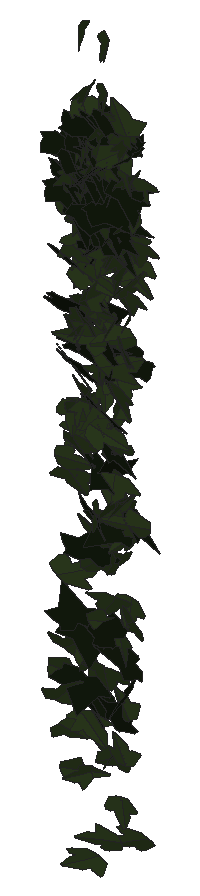
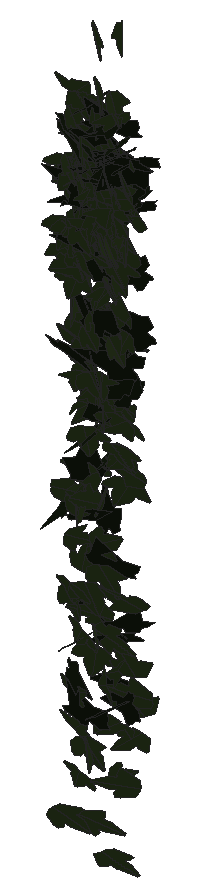
# SketchUp Ruby script. Lengths in millimetres.
U = 1.mm
M = Sketchup.active_model
def pt(a) = Geom::Point3d.new(a.map { |v| v * U })
def face(e, loops, mat)
  f = e.add_face(loops[0].map { |a| pt(a) })
  loops[1..].each { |l| e.add_face(l.map { |a| pt(a) }).erase! }
  f.material = f.back_material = mat if mat
  f
end
# faces: each face lists its corners as indices into pts; further lists are holes
def faces(e, pts, list, mat = nil) = list.each { |f| face(e, (f[0].is_a?(Array) ? f : [f]).map { |l| l.map { |i| pts[i] } }, mat) }
# xy, xz, yz: faces in a plane at the given z, y or x. An outline is a flat list of corners, or four numbers for a rectangle; further outlines are holes
def ring(l) = l.size == 4 ? [[l[0], l[1]], [l[2], l[1]], [l[2], l[3]], [l[0], l[3]]] : l.each_slice(2).to_a
def flat(e, list, mat, &to3) = list.each { |f| face(e, (f[0].is_a?(Array) ? f : [f]).map { |l| ring(l).map { |u, v| to3.(u, v) } }, mat) }
def xy(e, z, list, mat = nil) = flat(e, list, mat) { |x, y| [x, y, z] }
def xz(e, y, list, mat = nil) = flat(e, list, mat) { |x, z| [x, y, z] }
def yz(e, x, list, mat = nil) = flat(e, list, mat) { |y, z| [x, y, z] }
def lines(e, pts, list) = list.each { |a, b| e.add_line(pt(pts[a]), pt(pts[b])) }
# prism: a flat outline (further loops are holes) pulled along v
def prism(e, loops, v, mat = nil)
  f = face(e, loops, mat); d = Geom::Vector3d.new(v.map { |x| x * U })
  f.pushpull(f.normal.samedirection?(d) ? d.length : -d.length)
end
def box(e, o, s, mat = nil) = prism(e, [[o, [o[0] + s[0], o[1], o[2]], [o[0] + s[0], o[1] + s[1], o[2]], [o[0], o[1] + s[1], o[2]]]], [0, 0, s[2]], mat)
def at(x, y, z, deg = 0) = Geom::Transformation.translation(pt([x, y, z])) * Geom::Transformation.rotation(ORIGIN, Z_AXIS, deg.degrees)
def axes(o, x, y, z) = Geom::Transformation.new([*x, 0, *y, 0, *z, 0, *pt(o).to_a, 1])
def part(name) = M.definitions.add(name)
# library, detail: a bought-in or finely detailed component or shape, given as its bounding box
def library(name, o, s) = part(name).tap { |d| box(d.entities, o, s) }
def detail(e, o, s) = box(e.add_group.entities, o, s)
def put(e, d, t, mat = nil) = e.add_instance(d, t).tap { |i| i.material = mat if mat }
def group(e, t, mat = nil) = e.add_group.tap { |g| g.transformation = t; g.material = mat if mat }.entities
root = M.entities
M.materials.add("efeu1").color = [18, 25, 13]
M.materials.add("efeu2").color = [43, 57, 29]
c1 = part("ivyleaf_9")
p = [[39.1,54.8,31.7],[34.5,51.8,30.2],[-5.3,25.2,17.3],[-17.9,28.3,20.9],[-21.6,21.7,17],[-20.2,4.3,5.3],
  [-22.9,-0.3,2.5],[-17.1,-4,-0.6],[-2,-2.1,-1.2],[-0.7,-15.4,-10.1],[16.6,-22.3,-16.7],[21.1,-15.1,-12.5],
  [32.7,-10.7,-11],[46.1,-1.8,-6.6],[30.8,11.2,3.8]]
faces(c1.entities,p,[[0,1,2,3,4,5,6,7,8,9,10,11,12,13,14]],"efeu1")
c2 = part("ivyleaf_10")
p = [[0,12.8,-0.8],[-1.5,51.3,-10.9],[-4.9,51,-11.6],[-13.6,26.5,-7.3],[-13.2,15.9,-4.6],[-21.1,19.3,-7.2],
  [-29.5,16.3,-8.3],[-29.2,8.3,-6.2],[-19.7,-9.8,0.5],[-7.6,-13,4],[1,-12.2,5.8],[-0.4,51.1,-11.1],
  [-1.5,51.1,-10.9],[1,-12.4,5.9],[16.9,-12.4,3.5],[35.1,9.1,-5.1],[35,12.9,-6.1],[20.5,16.4,-4.9],
  [15.8,15,-3.8],[15.3,27.6,-7.1],[12.8,31.3,-7.8]]
faces(c2.entities,p,[[0,1,2,3,4,5,6,7,8,9,10],[11,12,0,13,14,15,16,17,18,19,20]],"efeu2")
put(root,c1,axes([1991.5,1004.4,1194.2],[0.3443,-0.71439,0.18817],[0.06555,-0.18537,-0.73684],[1.40447,0.18378,-0.01174]))
put(root,c1,axes([1980.8,1001,965],[1.26867,-0.16878,0.32157],[0.57945,-0.1067,-0.68714],[0.3768,0.73237,-0.026]))
put(root,c2,axes([2021.5,998.1,1111.6],[-0.50101,0.3868,0.60638],[-0.75739,0.45955,-0.4659],[-1.14025,-0.4752,0.04303]))
put(root,c2,axes([2009.7,1013.5,951.1],[-1.0539,0.40391,-0.02683],[0.05209,-0.008,-0.68534],[-0.76866,-0.55434,-0.00966]))
put(root,c2,axes([2015,1011.7,1198.3],[-0.38159,-0.68078,0.27221],[0.05991,-0.28994,-0.70193],[1.39412,-0.17388,0.10467]))
put(root,c2,axes([2013.6,1011.5,1227],[0.61604,-0.689,-0.06926],[0.01293,0.0796,-0.7602],[1.31784,0.3213,0.03983]))
put(root,c2,axes([1984.2,1000.6,322.6],[0.07398,0.0017,0.76415],[1.39024,0.22458,-0.03766],[-0.42702,0.73144,0.00979]))
put(root,c2,axes([2005.2,983.6,287.5],[-0.90609,-0.56331,0.27317],[0.33627,0.20834,0.73755],[-1.14306,0.50782,0.00044]))
put(root,c2,axes([1989.2,1014,486.7],[0.89653,0.00926,-0.62372],[1.15221,0.18157,0.45993],[0.28611,-0.76024,0.10225]))
put(root,c2,axes([2002.5,1002.3,365.7],[-1.16264,-0.11009,0.35684],[0.69416,-0.02903,0.61544],[-0.15256,0.70688,0.08084]))
put(root,c1,axes([1993.6,1018.7,854],[0.32542,-0.49134,0.58275],[0.33466,-0.5557,-0.52013],[1.41157,0.24502,-0.01103]))
put(root,c1,axes([1992.8,1004.3,1198.2],[0.97504,-0.54222,0.14142],[0.18744,-0.10151,-0.74597],[1.04988,0.52169,0.00184]))
put(root,c1,axes([1995,987.6,1060.5],[1.28577,-0.35581,0.01874],[0.03153,-0.00876,-0.76355],[0.67738,0.67579,-0.00003]))
put(root,c2,axes([2015.4,993.3,1199.4],[-0.19493,-0.76074,-0.06956],[0.24393,0.05208,-0.75823],[1.43327,-0.11233,0.11958]))
put(root,c1,axes([2004.2,992.4,1176.2],[-0.04385,-0.67202,-0.39365],[0.05034,0.39292,-0.67232],[1.48141,-0.03325,0.01119]))
put(root,c2,axes([2020.4,1026.9,941.7],[-0.03177,-0.70495,0.14492],[-0.02742,-0.1446,-0.70507],[1.36945,-0.01925,-0.01076]))
put(root,c2,axes([2010.7,995.7,938.7],[-0.56729,0.62076,-0.2373],[0.19812,-0.21325,-0.68862],[-1.2492,-0.31572,-0.00145]))
put(root,c1,axes([2005.9,992.9,1257.2],[-0.38579,-0.62426,-0.40755],[0.32536,0.37217,-0.65509],[1.38105,-0.26206,0.04048]))
put(root,c2,axes([2008.3,984.8,238.3],[-0.61775,-0.31187,-0.51603],[0.73211,0.34418,-0.44997],[0.88367,-0.50317,0.01205]))
put(root,c1,axes([2028.9,991.4,426.4],[-1.02894,-0.43395,0.31429],[0.54717,0.14181,0.69037],[-0.86052,0.60906,0.06318]))
put(root,c2,axes([2044,996.7,1127.8],[-0.6876,0.2033,0.63139],[-1.18847,0.1382,-0.40182],[-0.42571,-0.7142,0.10197]))
put(root,c2,axes([2026.4,1009.1,747.8],[1.22146,-0.18739,-0.23723],[-0.42712,0.07766,-0.6685],[0.38549,0.67981,0.01098]))
put(root,c2,axes([2019.8,993.1,678.7],[-1.30137,-0.15233,-0.18445],[0.34277,0.0398,-0.70054],[0.29964,-0.7071,0.0003]))
put(root,c2,axes([2015.2,1007.7,1201.8],[-0.95157,0.42483,-0.36369],[0.37239,-0.32413,-0.64761],[-0.99709,-0.52649,0.10522]))
put(root,c2,axes([2021,1018.7,1152.4],[0.92649,-0.56554,-0.00913],[0.11615,0.06449,-0.74096],[1.0702,0.4826,0.08831]))
put(root,c1,axes([1999.8,1010.3,310.2],[0.05461,0.00619,-0.79542],[1.50855,-0.06702,0.02807],[-0.12706,-0.79311,-0.00858]))
put(root,c1,axes([2010.6,1011.3,855.1],[1.27088,-0.3612,-0.15555],[0.26421,-0.0703,0.75917],[-0.70029,-0.68202,0.00413]))
put(root,c2,axes([1999.8,995.5,700],[0.27727,-0.08799,-0.68476],[1.17858,-0.29273,0.16937],[-0.58088,-0.63595,0.01678]))
put(root,c1,axes([2013,992,1241.4],[1.28017,0.41599,0.13611],[0.21094,0.07954,-0.79083],[-0.80586,0.68165,0.00921]))
put(root,c2,axes([2051.7,1010.3,414.8],[0.25022,-0.05893,-0.79799],[-1.23912,0.46223,-0.14141],[0.88527,0.66364,0.02762]))
put(root,c2,axes([2020.2,1016.5,1132.5],[-0.75795,0.55492,-0.26846],[0.27034,-0.2284,-0.68284],[-1.14165,-0.4225,0.01654]))
put(root,c2,axes([2017.9,994.7,792.6],[1.17273,-0.39934,0.27306],[0.42872,-0.15449,-0.73424],[0.81481,0.65604,-0.00668]))
put(root,c2,axes([2041.9,995.6,941],[-1.08903,0.42577,-0.3097],[-0.47097,0.18623,0.71324],[0.88445,0.62343,-0.00154]))
put(root,c2,axes([2021.9,998.5,736.9],[-1.16936,0.2705,-0.22588],[0.39418,-0.09015,-0.67132],[-0.54264,-0.64838,-0.0009]))
put(root,c2,axes([2028.1,1015.9,1073.6],[1.4453,0.06037,-0.11549],[-0.22025,-0.00152,-0.76176],[-0.11403,0.76813,0.00757]))
put(root,c2,axes([2009.7,999.8,156.5],[0.02876,-0.0893,0.72977],[0.88507,0.56652,0.05969],[-1.08378,0.46027,0.06811]))
put(root,c1,axes([2018.4,989.2,1239.4],[0.47847,-0.55105,-0.46574],[-0.2494,0.45013,-0.60332],[1.35034,0.27839,0.0536]))
put(root,c2,axes([2033.1,1022,1111.3],[0.25496,-0.72577,0.02753],[0.00931,-0.02709,-0.73803],[1.38225,0.13405,-0.00011]))
put(root,c2,axes([2030.7,1004.8,1043.2],[0.0591,-0.66909,0.33814],[0.21229,-0.33053,-0.66429],[1.4109,0.07776,0.08579]))
put(root,c2,axes([2029.4,1000,352.8],[0.09739,0.19029,-0.67696],[0.26729,0.66231,0.19679],[1.31136,-0.14913,0.01016]))
put(root,c2,axes([2006.2,992.6,1156.6],[0.74594,-0.11506,0.7151],[1.32334,-0.1679,-0.40812],[0.38598,0.798,0.01724]))
put(root,c2,axes([2050.2,1018.4,527.6],[-1.12574,-0.05811,0.38811],[-0.72852,-0.06929,-0.59376],[0.16462,-0.70406,0.0264]))
put(root,c2,axes([2036.5,996,939.5],[-0.04128,-0.71602,-0.0118],[0.01417,0.01158,-0.71631],[1.36283,-0.02181,0.00709]))
put(root,c2,axes([2021.4,1008.1,795.1],[-1.01232,0.07988,-0.40814],[0.73504,-0.15094,-0.53286],[-0.29363,-0.65324,0.07322]))
put(root,c2,axes([2042.9,997.1,162.1],[0.04607,0.02446,-0.67286],[-0.62464,-0.58746,-0.03316],[-1.11888,0.32897,-0.00919]))
put(root,c2,axes([2009.1,1020.3,1197.1],[0.73009,-0.0376,0.63466],[1.20997,0.02761,-0.38264],[-0.00805,0.74107,0.04646]))
put(root,c2,axes([2030.4,1015.4,1205.9],[0.61389,-0.64916,0.20141],[0.31888,-0.14011,-0.71994],[1.25365,0.35352,0.0845]))
put(root,c2,axes([2034.4,1005.2,1195.7],[0.41638,-0.65907,-0.30655],[0.16071,0.34102,-0.6729],[1.37402,0.15983,0.1716]))
put(root,c1,axes([2033.1,1005.8,1251.7],[-1.03708,-0.54449,-0.25806],[0.3469,0.18267,-0.77032],[1.09303,-0.57459,-0.00036]))
put(root,c2,axes([2039.4,1003.3,1354],[-0.0746,-0.77444,-0.07693],[0.00115,0.077,-0.77542],[1.48116,-0.03906,-0.00327]))
put(root,c2,axes([2045.7,1002,1117.9],[0.48998,-0.39341,-0.56744],[-0.44222,0.52092,-0.46658],[1.23748,0.34193,0.05795]))
put(root,c2,axes([2041.3,1007.1,983],[0.53009,-0.62264,-0.23066],[-0.20904,0.20348,-0.6819],[1.24629,0.29896,-0.01627]))
put(root,c1,axes([2005.9,1006,896.9],[0.67409,-0.04591,0.68883],[1.30732,-0.05393,-0.35679],[0.13129,0.77268,0.01602]))
put(root,c2,axes([2042,998.5,1136.1],[-0.16031,-0.69939,0.27486],[-0.0127,-0.27587,-0.70402],[1.43013,-0.08085,0.02456]))
put(root,c2,axes([2062.7,992.9,933.2],[0.57372,-0.00002,-0.75208],[-1.42767,-0.05807,-0.30067],[-0.10257,0.80816,-0.02162]))
put(root,c2,axes([2052.6,996.2,18],[0.86702,0.1131,-0.50583],[-0.95314,-0.07752,-0.46837],[-0.25425,0.67631,0.0309]))
put(root,c2,axes([2046.2,978.3,1466.7],[-0.25411,0.75234,0.29595],[-0.5932,0.22887,-0.72243],[-1.41971,-0.23029,0.24888]))
put(root,c2,axes([2032.8,1021.5,1166.6],[0.8995,0.56844,0.00239],[0.00355,0.00156,-0.73925],[-1.08185,0.47263,-0.00043]))
put(root,c2,axes([2032.9,997,794],[-0.64537,-0.65241,0.26453],[0.22286,0.23725,0.73526],[-1.32119,0.35871,-0.00519]))
put(root,c2,axes([2029.6,994.6,1260.8],[0.98153,-0.44161,0.32341],[0.4918,-0.19529,-0.67873],[0.91836,0.57657,0.01782]))
put(root,c2,axes([2042.1,1010.4,1216.6],[0.31069,-0.74617,0.0146],[0.01506,-0.01322,-0.7638],[1.42031,0.16336,0.0049]))
put(root,c2,axes([2033.1,1002.6,1323.9],[0.56994,0.75244,0.04328],[0.02961,0.04039,-0.80984],[-1.4341,0.29987,0.00048]))
put(root,c1,axes([2027.4,1005.2,1260.5],[0.1564,-0.76174,-0.10428],[-0.00567,0.10455,-0.76611],[1.46325,0.08183,0.00818]))
put(root,c2,axes([2032.4,989,1078.7],[-0.94116,-0.39185,-0.37432],[0.6714,0.15189,-0.62505],[0.78289,-0.60133,0.08604]))
put(root,c1,axes([2030,1028.7,296.8],[-0.06688,-0.79581,0.03387],[0.0023,-0.03395,-0.79658],[1.51595,-0.03505,0.0027]))
put(root,c1,axes([2028.3,998.4,1133],[0.09126,-0.71629,0.32908],[0.00609,-0.32951,-0.71769],[1.50023,0.04491,-0.0171]))
put(root,c2,axes([2039.7,1018.8,1037.2],[0.71655,-0.59287,0.16432],[0.14037,-0.14776,-0.70212],[1.16243,0.3833,-0.01651]))
put(root,c1,axes([2041.5,995,328.5],[-1.19031,-0.36181,-0.31053],[0.50423,0.16212,-0.72251],[0.75445,-0.67919,-0.00704]))
put(root,c2,axes([2045.3,1022.1,1111],[0.25255,-0.72563,-0.02654],[0.00446,0.02741,-0.73763],[1.38194,0.13252,0.00723]))
put(root,c2,axes([2062.5,1010,570.1],[-0.81961,0.32413,-0.49227],[-0.82884,0.23582,0.53626],[0.75585,0.61006,0.05426]))
put(root,c1,axes([2039.6,1009.2,534.9],[-1.13625,0.09361,0.49924],[0.87449,-0.22888,0.59239],[0.41208,0.74384,0.11945]))
put(root,c2,axes([2035.1,1000.4,818.6],[-0.83771,0.34897,0.46675],[0.70424,-0.28454,0.56169],[0.8569,0.57501,-0.00532]))
put(root,c1,axes([2039.3,1005.1,410.8],[-0.62571,-0.69901,-0.15551],[0.13886,0.13753,-0.77243],[1.35578,-0.33669,0.00734]))
put(root,c1,axes([2034.8,1010.8,1270.6],[0.01024,-0.7004,0.29604],[-0.00422,-0.29606,-0.70041],[1.44718,0.00409,-0.00414]))
put(root,c2,axes([2038.3,1020.6,1170.7],[1.36994,0.13529,0.10598],[0.1879,0.048,-0.73185],[-0.26772,0.72598,0.02864]))
put(root,c1,axes([2068,998.4,895.2],[0.21903,-0.18919,0.79245],[-0.87595,0.64529,0.2209],[-1.27947,-0.47416,-0.01557]))
put(root,c2,axes([2033.2,1027.4,336.8],[0.45309,-0.32545,0.65801],[0.95892,-0.43064,-0.39529],[1.01608,0.55154,0.07963]))
put(root,c2,axes([2062.2,1008.6,852.7],[-0.48151,0.3315,0.61469],[-0.72876,0.48091,-0.41696],[-1.11157,-0.45889,0.00709]))
put(root,c2,axes([2048.8,996.5,1146],[-0.03103,0.50336,0.57724],[0.00058,0.57738,-0.50347],[-1.45764,-0.01049,-0.01249]))
put(root,c1,axes([2046.9,975.3,1209],[0.51301,0.22076,0.68083],[0.59918,0.61679,-0.32463],[-1.22332,0.39467,0.12651]))
put(root,c1,axes([2043.1,1010.2,1205.1],[-0.23815,-0.67016,0.34329],[0.18746,-0.35958,-0.66605],[1.42073,-0.06489,0.14543]))
put(root,c1,axes([2049.2,1014.4,1050.6],[0.51504,0.45231,0.56893],[-0.56462,-0.48547,0.52707],[1.2628,-0.40154,0.00362]))
put(root,c2,axes([2056.1,987.3,804.7],[1.34547,-0.05943,-0.10901],[-0.20472,0.0216,-0.70933],[0.11801,0.71498,0.01236]))
put(root,c2,axes([2067.4,1021.1,862.7],[-0.93308,-0.429,0.20414],[-0.26031,-0.15347,-0.65101],[0.86591,-0.50841,0.02427]))
put(root,c1,axes([2047.1,1003.8,603.9],[-0.30176,0.00295,0.8534],[0.15977,-0.86374,0.01858],[1.61633,0.08593,0.15749]))
put(root,c2,axes([2038,997.9,256.2],[1.18749,0.13375,0.4526],[0.84391,0.09078,-0.63811],[-0.30757,0.76545,-0.00341]))
put(root,c2,axes([2061,990.5,1238.9],[0.07983,-0.65864,-0.47305],[0.09228,0.47487,-0.65688],[1.54057,0.00568,0.06386]))
put(root,c2,axes([2033.1,1000,972.8],[-0.38956,-0.18173,0.70751],[1.38801,-0.0093,0.20861],[-0.0786,0.73646,0.17722]))
put(root,c1,axes([2042.2,997.8,1311.2],[1.14181,-0.47201,-0.18385],[-0.18473,0.17259,-0.75982],[0.94622,0.60328,0.07352]))
put(root,c2,axes([2054.3,1010.4,1016.8],[0.16466,0.72593,0.09804],[0.03623,0.09646,-0.73103],[-1.39366,0.08827,-0.00742]))
put(root,c2,axes([2067,1011.1,1188.9],[0.5226,0.6496,-0.24477],[-0.63635,-0.10692,-0.65884],[-1.15783,0.35197,0.25162]))
put(root,c2,axes([2061.9,990.8,1274.4],[0.86492,-0.63197,0.01893],[0.0208,-0.01545,-0.77841],[1.20313,0.45458,-0.00015]))
put(root,c2,axes([2061.1,995.3,1014.9],[-0.4265,-0.56013,-0.4322],[0.27109,0.40836,-0.60308],[1.31892,-0.26506,-0.0158]))
put(root,c2,axes([2076.9,985.1,792.9],[-0.32641,0.19933,0.78904],[-0.93854,0.61602,-0.26281],[-1.23214,-0.52204,-0.00884]))
put(root,c2,axes([2065.1,997.8,1114],[0.02907,-0.7265,-0.18855],[0.03336,0.18888,-0.72636],[1.42809,0.01038,0.0208]))
put(root,c1,axes([2058.1,975.8,1214.7],[0.5515,0.39713,0.59081],[0.42604,0.55469,-0.48265],[-1.28612,0.35404,0.09346]))
put(root,c2,axes([2064.1,1015.5,1138.4],[-0.4712,-0.65102,-0.24879],[0.23239,0.21941,-0.69567],[1.30589,-0.27395,0.03403]))
put(root,c1,axes([2053.9,982.8,1286.7],[-0.82352,0.04813,0.67201],[1.25237,-0.14123,0.43381],[0.27521,0.78669,0.03677]))
put(root,c1,axes([2046.1,1020.5,958.9],[-0.1659,0.03371,0.78745],[0.84205,-0.65356,0.07696],[1.24141,0.44781,0.05303]))
put(root,c2,axes([2069.8,1029.4,946.8],[-0.17341,-0.67476,0.2638],[0.0924,-0.27097,-0.67632],[1.37576,-0.06685,0.07868]))
put(root,c2,axes([2069.1,1015.1,966.8],[-0.27213,-0.65516,0.24738],[0.17725,-0.26803,-0.65602],[1.32099,-0.099,0.13898]))
put(root,c2,axes([2071.9,974.8,1009.9],[-0.08216,0.05821,0.81046],[-0.39192,0.78432,-0.06731],[-1.49595,-0.20868,-0.02688]))
put(root,c2,axes([2061.2,1017.9,400.5],[0.04251,-0.08227,-0.73938],[0.20675,-0.73143,0.08467],[-1.4007,-0.11046,-0.00994]))
put(root,c1,axes([2062.1,1008.9,1230.7],[-0.29765,-0.75027,0.02733],[0.01024,-0.02903,-0.76632],[1.42882,-0.15609,0.01118]))
put(root,c1,axes([2089.5,1010.3,1192.4],[-1.432,-0.00849,0.10189],[-0.19395,0.00091,-0.75246],[0.01578,-0.75928,-0.00204]))
put(root,c1,axes([2088.3,998.4,890.1],[-0.20102,0.10538,-0.81586],[-1.34902,0.4058,0.14418],[0.79458,0.71562,0.03838]))
put(root,c2,axes([2082.8,1022.9,1069],[-1.25059,-0.14991,0.27901],[-0.36589,-0.32189,-0.62572],[0.47906,-0.63719,0.25045]))
put(root,c2,axes([2095.7,991.9,65.5],[-0.27759,-0.07919,0.66045],[-1.0786,-0.33921,-0.16583],[0.66281,-0.58516,0.00675]))
put(root,c2,axes([2068.5,1015.4,1186.5],[0.27775,0.73782,0.07411],[-0.03946,0.07956,-0.75127],[-1.41073,0.14304,0.0356]))
put(root,c2,axes([2070.8,1010.7,836.2],[0.34745,0.62411,-0.20624],[-0.12986,-0.1949,-0.65018],[-1.24423,0.19462,0.01027]))
put(root,c1,axes([2070.5,1006.3,695.2],[-0.33703,-0.46496,0.63976],[-0.28019,-0.62476,-0.49481],[1.47888,-0.22433,0.05205]))
put(root,c2,axes([2046.5,982.4,1044.4],[0.7179,0.16897,0.68103],[1.21559,0.23746,-0.41268],[-0.55293,0.74142,-0.02303]))
put(root,c2,axes([2094.1,1005.4,205.2],[-0.97906,0.03771,0.49433],[-0.94169,0.00559,-0.51534],[-0.05912,-0.71342,0.02209]))
put(root,c2,axes([2082.9,1007.8,1105.9],[-1.11339,-0.39711,0.13249],[-0.1816,-0.09519,-0.70663],[0.77576,-0.59222,0.02474]))
put(root,c1,axes([2101.6,986.8,426.2],[-0.5229,0.39585,0.58721],[-0.73405,0.44461,-0.48017],[-1.13037,-0.47184,0.04018]))
put(root,c2,axes([2079.6,991.6,1360.1],[0.6215,-0.65672,-0.3272],[-0.06593,0.34394,-0.7249],[1.39486,0.30887,0.11152]))
put(root,c2,axes([2051.8,999.2,1100.2],[0.1233,0.0345,0.76569],[1.18183,0.44807,-0.07273],[-0.85509,0.62426,0.00989]))
put(root,c2,axes([2083.5,1010.9,207.9],[0.11693,-0.60006,-0.46953],[-0.11711,0.46561,-0.6031],[1.44535,0.08627,-0.01088]))
put(root,c2,axes([2073.2,1011.2,1181.4],[0.67127,-0.65596,0.04882],[0.32395,0.03751,-0.72573],[1.20923,0.35409,0.16732]))
put(root,c2,axes([2077,975.5,636.5],[0.25739,-0.45684,-0.57237],[0.21037,0.58812,-0.44329],[1.37781,-0.00445,0.17461]))
put(root,c2,axes([2090.7,1004.6,477.8],[-1.14474,-0.31617,0.2329],[-0.39008,-0.11063,-0.67951],[0.6375,-0.63544,0.00242]))
put(root,c2,axes([2086.6,1020.8,1113.9],[-0.71703,-0.61699,0.15743],[-0.1349,-0.14115,-0.72281],[1.20434,-0.38314,0.01277]))
put(root,c2,axes([2081.4,1000,1081.2],[-0.30091,-0.6558,0.34889],[0.17427,-0.37119,-0.65622],[1.40297,-0.09455,0.15634]))
put(root,c2,axes([2104.7,1011.9,1162.3],[-0.79078,0.1747,-0.59545],[-1.1123,0.13072,0.44617],[0.397,0.71422,0.06399]))
put(root,c2,axes([2082.4,992.5,1225.9],[-1.20489,-0.38631,-0.09643],[0.20684,0.00658,-0.73992],[0.72902,-0.64035,0.05057]))
put(root,c2,axes([2085.7,1017.5,1197.1],[-1.07822,0.46554,0.14458],[-0.21936,0.08746,-0.73325],[-0.90146,-0.57811,0.00549]))
put(root,c1,axes([2055,993,1081.4],[0.61384,0.05696,0.7663],[1.38486,0.24446,-0.32443],[-0.47002,0.79466,0.04487]))
put(root,c2,axes([2083.7,985.4,1308.7],[-0.1516,-0.73738,-0.25761],[0.12994,0.25138,-0.74067],[1.48087,-0.09754,0.03862]))
put(root,c2,axes([2083.7,991.8,1453.5],[0.67413,-0.69697,-0.18728],[0.01253,0.21173,-0.77552],[1.37346,0.34016,0.099]))
put(root,c1,axes([2093.4,995.5,1127],[-0.84537,0.56272,-0.38659],[0.47195,-0.29673,-0.71684],[-1.21061,-0.50862,-0.0095]))
put(root,c2,axes([2071.4,1016.1,692.6],[-0.80432,0.38138,-0.38604],[0.55906,-0.25063,-0.56919],[-0.86839,-0.5146,-0.00888]))
put(root,c2,axes([2087.7,988.6,361.2],[-1.39854,0.04403,0.0393],[-0.07534,-0.00361,-0.73613],[-0.08331,-0.73588,0.00596]))
put(root,c1,axes([2079.1,1015.1,690],[0.79212,0.40639,0.59318],[-0.83918,-0.39714,0.58146],[1.08096,-0.60611,0.01673]))
put(root,c2,axes([2086.4,996.1,1197.6],[0.6528,-0.67087,-0.24637],[-0.08009,0.25384,-0.7498],[1.35782,0.33751,0.07422]))
put(root,c2,axes([2087,1013.7,1191.8],[-1.382,0.21839,0.02958],[-0.05904,-0.00044,-0.75822],[-0.41525,-0.72675,0.00935]))
put(root,c2,axes([2085,1012.1,1120.6],[0.8844,-0.57091,-0.03736],[-0.03946,0.0313,-0.73611],[1.08816,0.46514,0.00367]))
put(root,c1,axes([2054.9,998.8,804.6],[1.02695,-0.10676,-0.6499],[1.20759,-0.14097,0.54997],[-0.33604,-0.83286,-0.00978]))
put(root,c2,axes([2085.2,1024.2,531.8],[-0.24999,-0.56196,-0.43447],[-0.21717,-0.41941,0.57697],[-1.33433,0.17354,-0.0125]))
put(root,c2,axes([2064.6,997.1,435],[-0.21345,-0.08152,0.65502],[0.95931,0.4184,0.13837],[-0.8111,0.5163,-0.00871]))
put(root,c1,axes([2096.2,1007.9,609.1],[-1.00811,-0.47413,0.28475],[-0.38137,-0.20296,-0.71071],[0.98107,-0.56609,0.01632]))
put(root,c2,axes([2072.5,1021.4,1126.5],[-1.05414,-0.24517,-0.41694],[0.88902,-0.10668,-0.55781],[0.23883,-0.68501,0.23609]))
put(root,c1,axes([2074.9,1001.4,1123.1],[0.2927,-0.64621,-0.38759],[-0.05119,0.39062,-0.66193],[1.43321,0.14593,0.05551]))
put(root,c2,axes([2085.1,997.4,627.9],[0.12628,-0.43948,0.72964],[-0.07306,0.72956,0.44293],[-1.61945,-0.06718,0.03691]))
put(root,c1,axes([2075.6,1017.7,259.3],[-0.66504,0.15803,0.67847],[0.79572,-0.55957,0.34567],[1.06051,0.51896,0.16611]))
put(root,c2,axes([2096.9,1001.7,749.2],[-0.9688,-0.44696,0.07923],[-0.10499,-0.05725,-0.67738],[0.85751,-0.51197,0.00658]))
put(root,c1,axes([2063.4,978.3,1167.6],[0.49611,-0.27434,-0.85378],[0.54661,0.86783,-0.19116],[1.61684,-0.20921,0.3266]))
put(root,c2,axes([2092.1,1011,1260.6],[0.09085,-0.72337,-0.23496],[0.10124,0.23802,-0.72199],[1.44397,0.02882,0.0654]))
put(root,c2,axes([2108.2,1007.5,941.7],[-0.4199,-0.17164,0.69378],[-0.63407,-0.61767,-0.25876],[1.20338,-0.38535,0.10574]))
put(root,c2,axes([2104.7,987.8,1269.6],[1.29213,-0.09891,-0.43903],[-0.82465,0.07104,-0.68606],[0.23143,0.80538,0.0066]))
put(root,c2,axes([2095.1,993.7,969.8],[0.44839,-0.73119,-0.00605],[-0.00304,0.00584,-0.76821],[1.39165,0.2356,0.00027]))
put(root,c1,axes([2080.4,999.6,753.7],[0.76786,-0.57241,-0.32294],[-0.31659,0.27766,-0.69997],[1.21011,0.43586,0.02179]))
put(root,c1,axes([2086.7,1005.6,1278],[-0.78507,-0.54509,-0.36487],[0.43601,0.28415,-0.68351],[1.16977,-0.47174,0.00989]))
put(root,c2,axes([2098.8,1010.2,1079.9],[-0.47932,-0.68607,-0.04226],[-0.01441,0.04777,-0.73045],[1.30811,-0.25086,-0.02353]))
put(root,c2,axes([2096.8,1022.4,1071.8],[0.43872,-0.68202,-0.07062],[-0.00562,0.07352,-0.71963],[1.30494,0.22961,0.02064]))
put(root,c2,axes([2098.8,1031.7,578.9],[-0.23036,-0.29918,0.64305],[0.0082,-0.65265,-0.30283],[1.3498,-0.04709,0.11158]))
put(root,c1,axes([2069.1,1005,1177.1],[0.92545,0.59301,-0.2851],[0.35303,0.21657,0.76687],[1.20149,-0.52041,-0.00573]))
put(root,c2,axes([2096,1023.6,624.8],[-0.24119,-0.53979,-0.46269],[-0.23653,-0.44593,0.55427],[-1.33225,0.17689,-0.01464]))
put(root,c2,axes([2089.2,1012.1,1147.2],[-0.20288,-0.48141,0.55439],[0.5383,-0.54389,-0.41791],[1.28956,0.1513,0.26167]))
put(root,c2,axes([2098.1,1012.8,1215],[0.34967,-0.73548,-0.03494],[0.01015,0.03734,-0.75795],[1.40131,0.18325,0.01421]))
put(root,c2,axes([2078.2,987.9,1120.6],[-0.87854,0.35338,-0.58612],[0.88397,-0.35751,-0.58135],[-0.9567,-0.65484,0.00108]))
put(root,c1,axes([2105.1,1012.1,1212.5],[-1.27848,-0.3612,-0.01235],[0.02138,0.00519,-0.76271],[0.68751,-0.67185,0.00075]))
put(root,c2,axes([2102,1008.7,1096.9],[0.16152,0.5669,-0.472],[-0.49593,-0.42144,-0.55304],[-1.31343,0.22885,0.15077]))
put(root,c2,axes([2096.7,1014.8,811.3],[0.17057,0.41437,-0.55894],[-0.18973,-0.5501,-0.4238],[-1.31055,0.13357,-0.01139]))
put(root,c1,axes([2082.7,987.9,1332.2],[0.76688,-0.55665,-0.39636],[-0.23649,0.39278,-0.67795],[1.27887,0.40643,0.11231]))
put(root,c2,axes([2087.6,1029.1,612.6],[-0.51097,0.27606,0.61112],[0.74914,-0.46807,0.38436],[1.03325,0.47588,0.02354]))
put(root,c2,axes([2094.8,997.9,691.3],[1.35055,0.20851,-0.02329],[-0.04577,-0.00075,-0.7396],[-0.39667,0.71,0.00606]))
put(root,c2,axes([2086.3,972.3,787.9],[0.40672,0.57914,0.6447],[0.3796,0.61332,-0.61706],[-1.60508,0.2918,0.01743]))
put(root,c2,axes([2098,1010.2,1231.1],[0.97483,-0.5653,-0.05899],[0.11467,0.13296,-0.75106],[1.07562,0.49815,0.13353]))
put(root,c2,axes([2110.6,989.2,1323.6],[1.23339,-0.02833,-0.40706],[-0.68355,0.323,-0.59427],[0.36859,0.69379,0.26004]))
put(root,c2,axes([2092.8,1009.6,855.5],[0.74781,0.54626,0.12166],[0.12301,0.10336,-0.67285],[-1.05799,0.39813,0.00776]))
put(root,c2,axes([2106.5,988.7,1039.9],[0.3749,-0.64033,-0.29423],[-0.13307,0.28624,-0.66975],[1.33455,0.20842,0.01587]))
put(root,c2,axes([2105.7,1013.9,1131.2],[-0.26203,-0.70978,-0.15906],[0.05082,0.15684,-0.723],[1.38342,-0.1402,-0.00357]))
put(root,c2,axes([2117,1006.8,288.3],[0.82173,-0.20389,0.53418],[-0.91949,0.2279,0.47748],[-0.58198,-0.64795,-0.00015]))
put(root,c2,axes([2101.7,995.3,634.1],[0.18904,-0.44647,0.64173],[-0.15714,0.63728,0.45615],[-1.47953,-0.12473,0.03355]))
put(root,c2,axes([2089.4,1015.7,406.1],[1.01491,-0.32469,0.41377],[0.70782,-0.18386,-0.6236],[0.7078,0.64944,0.03032]))
put(root,c1,axes([2092.8,978.7,1177.6],[-0.00893,-0.3709,-0.69976],[0.06994,0.69891,-0.3707],[1.50567,-0.03466,0.01307]))
put(root,c1,axes([2090.2,995,1114],[0.50418,-0.68887,-0.20091],[-0.06668,0.20149,-0.73706],[1.36405,0.26447,0.03823]))
put(root,c2,axes([2109,990.9,1136.4],[0.17532,-0.74944,-0.06245],[-0.00107,0.06285,-0.75505],[1.43128,0.09185,0.00709]))
put(root,c1,axes([2091,1011.8,1208],[0.26907,-0.74677,-0.04956],[0.03945,0.05432,-0.75943],[1.42383,0.13961,0.03041]))
put(root,c1,axes([2121.6,1008.1,1263.5],[-0.1445,0.52294,0.5575],[-0.14817,0.55204,-0.52842],[-1.4472,-0.10873,-0.00156]))
put(root,c2,axes([2112.8,1014.3,1197.6],[-0.62498,-0.67339,0.09079],[-0.01503,-0.09705,-0.74836],[1.2931,-0.32659,0.03518]))
put(root,c2,axes([2112.1,1011.4,978.3],[0.1608,-0.49569,-0.54792],[-0.05881,0.54864,-0.5011],[1.40498,0.0797,0.04174]))
put(root,c1,axes([2118.4,1015.7,373.2],[0.00833,-0.74572,-0.21046],[0.05186,-0.21019,0.74531],[-1.47378,-0.01161,0.02503]))
put(root,c2,axes([2111.5,1007.1,1017.9],[-1.2681,0.22065,-0.00081],[0.00054,-0.00172,-0.70188],[-0.41994,-0.6663,0.00154]))
put(root,c1,axes([2115.5,1011.3,328.4],[-0.72627,0.41646,-0.52655],[0.69311,-0.3804,-0.56479],[-1.07336,-0.52742,-0.00842]))
put(root,c2,axes([2114.6,983.5,1319.6],[1.23838,-0.35549,-0.26657],[-0.2852,0.26945,-0.72509],[0.79611,0.6495,0.15491]))
put(root,c2,axes([2110.9,998.7,1060.3],[0.28332,-0.65289,0.25509],[0.19738,-0.2374,-0.66812],[1.31937,0.17571,0.04518]))
put(root,c2,axes([2104.9,986.1,859.5],[-1.09347,0.52626,-0.26037],[0.37068,-0.17284,-0.77912],[-1.05419,-0.60665,-0.00389]))
put(root,c1,axes([2130.8,994.3,1275.8],[-0.51808,0.69051,0.18515],[-0.15839,0.16617,-0.74206],[-1.35136,-0.2842,0.01599]))
put(root,c1,axes([2127.1,1021.8,901.8],[-1.43146,0.10885,-0.11708],[0.21984,-0.01931,-0.75997],[-0.21034,-0.76095,0.00254]))
put(root,c2,axes([2121.2,991.3,218.2],[1.05459,-0.1744,0.3643],[-0.66003,0.11159,0.58091],[-0.39403,-0.65369,0.00197]))
put(root,c2,axes([2112.6,990.4,1091.4],[-0.1528,-0.65111,-0.29642],[0.24187,0.28056,-0.65069],[1.33992,-0.1249,0.08365]))
put(root,c2,axes([2132,996.7,456.5],[-0.88917,0.29563,0.57155],[-0.95271,0.27684,-0.55238],[-0.76953,-0.68433,0.02345]))
put(root,c2,axes([2131.2,997.5,1168.9],[0.66005,-0.3359,-0.57591],[-0.81249,0.38674,-0.48265],[0.97462,0.54989,-0.01234]))
put(root,c1,axes([2110.5,985.4,1140.9],[0.63413,-0.39721,-0.66676],[-0.74984,0.5386,-0.51774],[1.27262,0.51527,0.02718]))
put(root,c2,axes([2135.4,1012.9,72.5],[-0.62309,-0.2576,0.55576],[-0.84583,-0.33377,-0.41651],[0.8023,-0.55195,-0.0075]))
put(root,c2,axes([2120,1010.8,1222.4],[-0.1356,-0.75951,0.00136],[0.00085,-0.00141,-0.76285],[1.44551,-0.07125,0.00058]))
put(root,c2,axes([2090,993.7,891.9],[1.02681,-0.02131,-0.63672],[1.20916,-0.04373,0.5398],[-0.0897,-0.83342,-0.01204]))
put(root,c2,axes([2123.8,1015.7,1073.1],[0.88164,0.44904,-0.34316],[-0.58965,-0.16931,-0.63979],[-0.89956,0.55107,0.08305]))
put(root,c2,axes([2115.3,1011.9,1108],[-0.85375,-0.53531,-0.31249],[0.42276,0.22128,-0.69795],[1.10134,-0.49991,0.02568]))
put(root,c2,axes([2122.3,985.3,936.8],[-0.83013,0.60527,0.23711],[-0.27775,0.18707,-0.74601],[-1.20561,-0.45986,0.00861]))
put(root,c2,axes([2112.9,1012.3,477],[1.23913,-0.31542,0.15064],[0.26179,-0.06158,-0.72344],[0.61158,0.66543,0.00446]))
put(root,c2,axes([2130.4,981.2,1326.4],[1.30439,-0.10734,0.38785],[-0.71745,0.09688,0.69296],[-0.26809,-0.78152,0.03263]))
put(root,c2,axes([2114.3,991.7,1027.3],[0.0951,-0.69827,0.35422],[0.1608,0.35768,0.69317],[-1.48147,-0.006,0.09798]))
put(root,c2,axes([2125.4,1008.8,1107.6],[-1.45484,-0.05124,-0.02921],[0.05543,0.00226,-0.76613],[0.09761,-0.76497,-0.0003]))
put(root,c2,axes([2109.9,1000.1,1241.9],[0.34198,-0.6482,0.33945],[0.77374,-0.20217,-0.60127],[1.15784,0.32655,0.30154]))
put(root,c2,axes([2146.2,995.7,628.7],[0.01401,0.01589,0.74245],[-1.09073,-0.47205,0.01578],[0.89881,-0.5731,0.00758]))
put(root,c2,axes([2119.9,1009.1,1216.5],[-1.34584,-0.14617,-0.21647],[0.41909,0.00238,-0.72096],[0.26736,-0.73953,0.04046]))
put(root,c2,axes([2127.6,993.5,1296.4],[-0.10586,-0.77626,0.0687],[0.03892,-0.0703,-0.77784],[1.48265,-0.05358,0.02532]))
put(root,c1,axes([2115.7,1007.5,1202.7],[-0.18219,-0.76291,0.03566],[-0.0176,-0.03478,-0.76887],[1.45344,-0.09605,-0.00484]))
put(root,c2,axes([2101.5,1023.3,1046],[0.84548,-0.04921,0.57248],[1.09279,0.01099,-0.44462],[0.04085,0.72454,0.04562]))
put(root,c1,axes([2113.7,1015.4,627.8],[0.97049,-0.52739,-0.44858],[-0.56326,0.33762,-0.73336],[1.19126,0.58929,0.0187]))
put(root,c2,axes([2113.6,990.4,137.8],[1.10747,-0.21823,0.28683],[0.50933,-0.10322,-0.62147],[0.45943,0.64049,-0.00243]))
